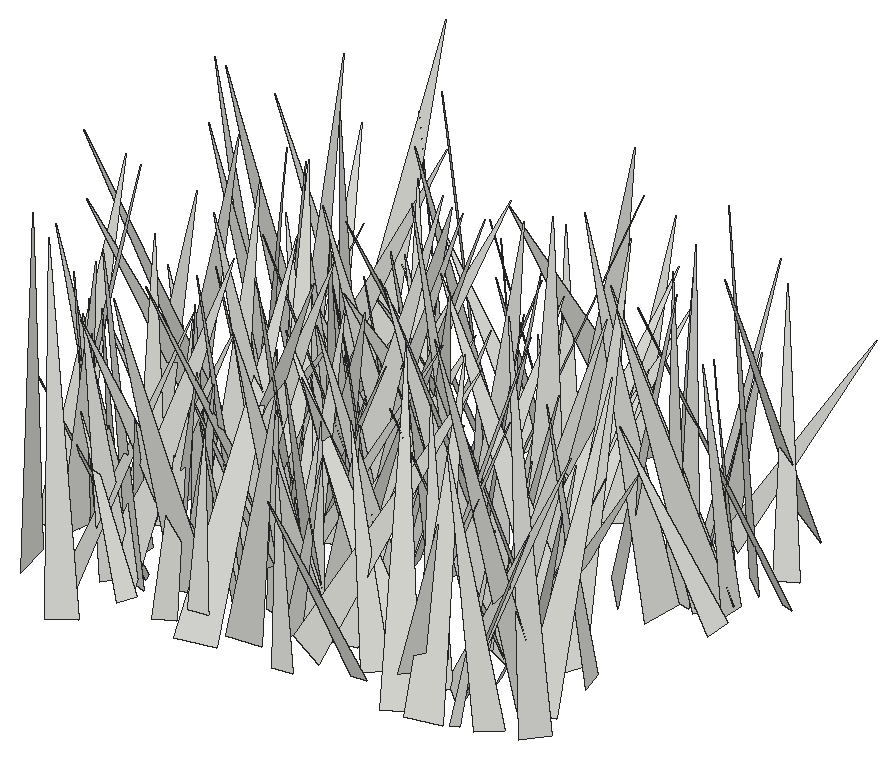
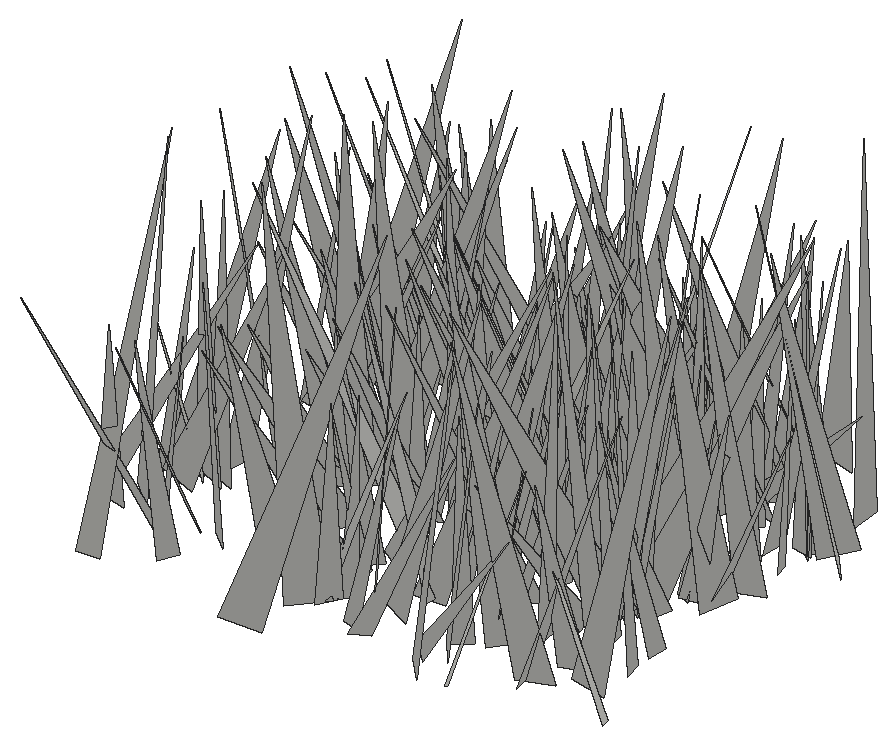
# SketchUp Ruby script. Lengths in inches.
U = 1.inch
M = Sketchup.active_model
def pt(a) = Geom::Point3d.new(a.map { |v| v * U })
def face(e, loops, mat)
  f = e.add_face(loops[0].map { |a| pt(a) })
  loops[1..].each { |l| e.add_face(l.map { |a| pt(a) }).erase! }
  f.material = f.back_material = mat if mat
  f
end
# faces: each face lists its corners as indices into pts; further lists are holes
def faces(e, pts, list, mat = nil) = list.each { |f| face(e, (f[0].is_a?(Array) ? f : [f]).map { |l| l.map { |i| pts[i] } }, mat) }
# xy, xz, yz: faces in a plane at the given z, y or x. An outline is a flat list of corners, or four numbers for a rectangle; further outlines are holes
def ring(l) = l.size == 4 ? [[l[0], l[1]], [l[2], l[1]], [l[2], l[3]], [l[0], l[3]]] : l.each_slice(2).to_a
def flat(e, list, mat, &to3) = list.each { |f| face(e, (f[0].is_a?(Array) ? f : [f]).map { |l| ring(l).map { |u, v| to3.(u, v) } }, mat) }
def xy(e, z, list, mat = nil) = flat(e, list, mat) { |x, y| [x, y, z] }
def xz(e, y, list, mat = nil) = flat(e, list, mat) { |x, z| [x, y, z] }
def yz(e, x, list, mat = nil) = flat(e, list, mat) { |y, z| [x, y, z] }
def lines(e, pts, list) = list.each { |a, b| e.add_line(pt(pts[a]), pt(pts[b])) }
# prism: a flat outline (further loops are holes) pulled along v
def prism(e, loops, v, mat = nil)
  f = face(e, loops, mat); d = Geom::Vector3d.new(v.map { |x| x * U })
  f.pushpull(f.normal.samedirection?(d) ? d.length : -d.length)
end
def box(e, o, s, mat = nil) = prism(e, [[o, [o[0] + s[0], o[1], o[2]], [o[0] + s[0], o[1] + s[1], o[2]], [o[0], o[1] + s[1], o[2]]]], [0, 0, s[2]], mat)
def at(x, y, z, deg = 0) = Geom::Transformation.translation(pt([x, y, z])) * Geom::Transformation.rotation(ORIGIN, Z_AXIS, deg.degrees)
def axes(o, x, y, z) = Geom::Transformation.new([*x, 0, *y, 0, *z, 0, *pt(o).to_a, 1])
def part(name) = M.definitions.add(name)
# library, detail: a bought-in or finely detailed component or shape, given as its bounding box
def library(name, o, s) = part(name).tap { |d| box(d.entities, o, s) }
def detail(e, o, s) = box(e.add_group.entities, o, s)
def put(e, d, t, mat = nil) = e.add_instance(d, t).tap { |i| i.material = mat if mat }
def group(e, t, mat = nil) = e.add_group.tap { |g| g.transformation = t; g.material = mat if mat }.entities
root = M.entities
c1 = part("fur_instance\#9")
p = [[0.8125,0,1.79],[0.67,-0.02,1.48],[0,-0.11,0],[0,0.11,0]]
faces(c1.entities,p,[[0,1,2,3]])
put(root,c1,axes([105.45,343.01,-27.1],[-1.01525,-4.25558,0.24661],[-4.20456,0.95799,-0.77812],[-0.70176,0.41691,4.30525]))
put(root,c1,axes([100.4375,342.52,-27.1],[2.54415,-5.74451,1.38415],[-5.89364,-2.3587,1.04378],[0.42454,1.68081,6.19537]))
put(root,c1,axes([94.2,339.64,-27.1],[-0.66678,7.09806,0.59701],[6.83624,0.46921,2.05647],[-2.00116,-0.76214,6.82627]))
put(root,c1,axes([102.92,341.7,-27.1],[-0.42877,3.87256,1.55947],[4.17346,0.35848,0.25729],[-0.1042,-1.57711,3.88772]))
put(root,c1,axes([90.58,342.37,-27.1],[7.19679,1.10507,2.93039],[1.40985,-7.70082,-0.55845],[-2.79655,-1.03845,7.25969]))
put(root,c1,axes([107.81,342.85,-27.1],[2.67886,-4.09104,0.57639],[-4.11516,-2.58128,0.80469],[0.36641,0.91951,4.82342]))
put(root,c1,axes([98.91,341.69,-27.1],[-3.06481,2.41196,1.362],[2.48233,3.29293,-0.24563],[1.22908,-0.63618,3.89234]))
put(root,c1,axes([96.72,344.24,-27.1],[1.44091,-6.85532,1.40735],[-6.89305,-1.6385,-0.92385],[-1.20912,1.1714,6.94393]))
put(root,c1,axes([95.12,342.3,-27.1],[-3.33504,1.53851,0.16438],[1.54705,3.32218,0.29368],[0.02564,-0.33558,3.66104]))
put(root,c1,axes([93.9,343.26,-27.1],[3.52477,-3.78027,2.43443],[-3.94318,-4.08529,-0.63451],[-2.1606,1.28874,5.1295]))
put(root,c1,axes([101.61,344.98,-27.1],[2.47706,-6.70826,1.39737],[-6.69174,-2.68793,-1.04158],[-1.47445,0.92925,7.07472]))
put(root,c1,axes([111.7,342.9,-27.1],[-2.10663,5.00928,1.58804],[5.23429,1.84857,1.1125],[-0.46582,-1.88217,5.31913]))
put(root,c1,axes([96.63,345.06,-27.1],[1.14957,-5.99203,1.40359],[-5.68779,-1.57972,-2.08556],[-2.35023,0.89221,5.73379]))
put(root,c1,axes([92.61,342.17,-27.1],[3.5807,5.01538,0.32607],[5.01642,-3.54168,-0.61141],[0.30977,-0.61982,6.13202]))
put(root,c1,axes([101.18,345.96,-27.1],[-2.08812,-6.42397,1.05341],[-6.15561,2.30841,1.87538],[2.11792,0.37569,6.48927]))
put(root,c1,axes([109.32,341.97,-27.1],[-1.91608,6.79372,1.10059],[6.8739,1.94553,-0.04218],[0.33984,-1.04766,7.05863]))
put(root,c1,axes([108.16,342.05,-27.1],[-2.69969,6.39263,0.77147],[6.43614,2.65406,0.5304],[-0.19237,-0.91623,6.91901]))
put(root,c1,axes([93.44,345.32,-27.1],[4.01305,-1.4697,0.35123],[-1.33059,-3.90931,-1.15533],[-0.71618,-0.97223,4.11458]))
put(root,c1,axes([94.71,343.38,-27.1],[-3.5063,-5.04513,2.56803],[-5.65565,3.25438,-1.32851],[0.24851,2.88062,5.99854]))
put(root,c1,axes([101.58,343.97,-27.1],[3.83893,-0.81047,1.08867],[-0.8917,-3.9684,0.19003],[-1.0232,0.41758,3.91895]))
put(root,c1,axes([109.6,343.875,-27.1],[4.10602,0.97464,0.35289],[0.9844,-4.11806,-0.08026],[-0.32469,-0.15985,4.21935]))
put(root,c1,axes([112.16,344.88,-27.1],[-1.47229,-7.46087,2.3597],[-7.72207,0.99683,-1.66627],[-1.2659,2.59656,7.41996]))
put(root,c1,axes([99.125,343.92,-27.1],[0.98464,3.25356,1.70885],[3.23357,-1.6077,1.19779],[-1.74639,-1.14237,3.18127]))
put(root,c1,axes([106.38,344.59,-27.1],[5.98331,3.57339,0.75673],[3.63565,-5.68637,-1.89446],[0.35186,-2.00943,6.70672]))
put(root,c1,axes([110.46,342.42,-27.1],[1.53322,3.39,0.04746],[3.12816,-1.43461,1.41479],[-1.30727,0.54307,3.44111]))
put(root,c1,axes([97.125,342,-27.1],[-5.33411,1.7362,0.45715],[1.45522,5.02033,-2.08679],[1.05153,1.85957,5.20696]))
put(root,c1,axes([108.97,344.19,-27.1],[3.86219,5.07234,0.99731],[5.04282,-3.42294,-2.11973],[1.1372,-2.04809,6.01264]))
put(root,c1,axes([105.66,343.76,-27.1],[-2.79772,3.91125,0.86225],[4.00509,2.73873,0.57209],[0.02536,-1.03446,4.77471]))
put(root,c1,axes([93.96,343.125,-27.1],[-0.17372,7.00266,1.70424],[6.95108,0.61311,-1.81067],[1.90374,-1.5996,6.76675]))
put(root,c1,axes([94.68,344.08,-27.1],[-3.03964,-3.22245,0.08473],[-2.53096,2.3136,-2.80576],[-1.9964,1.97328,3.42802]))
put(root,c1,axes([90.39,345.17,-27.1],[5.9168,-1.45412,1.7202],[-1.44139,-6.15974,-0.24915],[-1.73089,0.15879,6.08776]))
put(root,c1,axes([94.91,345.29,-27.1],[4.77554,-0.30271,1.03368],[-0.19329,-4.86277,-0.53104],[-1.0596,-0.47722,4.75556]))
put(root,c1,axes([108.18,344.16,-27.1],[2.13883,-4.28297,3.06723],[-5.00629,-2.68295,-0.2554],[-1.63976,2.60467,4.7805]))
put(root,c1,axes([108.15,344.68,-27.1],[3.13012,3.09581,1.75638],[3.35561,-3.34662,-0.08138],[-1.18695,-1.29717,4.40172]))
put(root,c1,axes([97.67,348.37,-27.1],[-5.6893,-5.57398,0.54513],[-5.22917,5.56506,2.3282],[2.00554,-1.30211,7.61688]))
put(root,c1,axes([102.64,343.47,-27.1],[1.86343,6.88556,0.79652],[6.51007,-1.45535,-2.64927],[2.37997,-1.41024,6.62304]))
put(root,c1,axes([90.87,345.73,-27.1],[-1.22041,-5.00142,1.71972],[-5.19067,1.47111,0.5948],[1.01418,1.51086,5.11369]))
put(root,c1,axes([102.03,344.65,-27.1],[3.56835,-1.26097,2.05366],[-1.59686,-3.9854,0.32755],[-1.80488,1.03305,3.77039]))
put(root,c1,axes([90.8,345.67,-27.1],[-3.25997,-4.21096,1.97124],[-4.4396,3.53441,0.20814],[1.38129,1.42168,5.3213]))
put(root,c1,axes([99.1,341.35,-27.1],[-6.13074,4.86156,0.06985],[4.48302,5.69573,-2.94734],[1.88206,2.26926,7.24803]))
put(root,c1,axes([100.23,345.47,-27.1],[-2.15609,-3.98258,0.83043],[-3.73233,1.56246,-2.1972],[-1.61872,1.70208,3.96005]))
put(root,c1,axes([93.35,344.57,-27.1],[2.79379,4.96818,0.70977],[4.95175,-2.59669,-1.31495],[0.8165,-1.25148,5.54607]))
put(root,c1,axes([91.86,346.13,-27.1],[-6.39617,-0.72322,1.67284],[-0.5993,6.59982,0.56183],[1.72113,-0.38959,6.41236]))
put(root,c1,axes([107.12,343.62,-27.1],[5.77926,4.78065,0.80242],[4.74367,-5.8345,0.5954],[-0.99801,-0.04845,7.47663]))
put(root,c1,axes([95.08,346.52,-27.1],[3.8804,-2.67072,0.47699],[-2.66948,-3.90717,-0.15997],[-0.48385,0.13783,4.70793]))
put(root,c1,axes([97.56,346.22,-27.1],[-5.57513,-2.9786,1.92177],[-3.03694,5.86084,0.2736],[1.82819,0.65252,6.315]))
put(root,c1,axes([106.45,344.64,-27.1],[-3.37764,5.82202,0.02709],[5.22944,3.02002,2.9728],[-2.55923,-1.51283,6.03878]))
put(root,c1,axes([113.3,343.6,-27.1],[-7.7657,1.30292,0.44128],[1.14319,7.51969,-2.08465],[0.76515,1.98873,7.59328]))
put(root,c1,axes([99.93,344.89,-27.1],[1.9045,4.44389,1.45881],[4.34306,-2.26488,1.22946],[-1.73613,-0.79091,4.67587]))
put(root,c1,axes([103.48,344.67,-27.1],[-2.78361,3.37072,1.19614],[3.02117,3.0272,-1.49988],[1.91443,0.12385,4.10617]))
put(root,c1,axes([94.83,347.07,-27.1],[-1.17903,-5.46423,1.73554],[-5.62366,1.44698,0.7353],[1.11548,1.51937,5.54141]))
put(root,c1,axes([108.22,347.99,-27.1],[-4.1053,-4.23157,0.31859],[-4.21802,4.11764,0.33835],[0.46467,-0.00766,5.88602]))
put(root,c1,axes([90.63,347.24,-27.1],[4.23333,1.58778,2.03705],[2.11026,-4.38143,-0.97034],[-1.48911,-1.69519,4.41595]))
put(root,c1,axes([99.28,346.92,-27.1],[1.07794,-7.21694,3.00432],[-7.53412,-1.768,-1.54384],[-2.08502,2.65746,7.13181]))
put(root,c1,axes([109.78,347.77,-27.1],[4.97063,-0.22915,0.23226],[-0.15729,-4.7897,-1.3593],[-0.28585,-1.34904,4.78665]))
put(root,c1,axes([89.03,345.81,-27.1],[-4.56158,-4.36485,4.54967],[-5.17144,5.80258,0.38189],[3.60662,2.79958,6.30192]))
put(root,c1,axes([100.9375,347.31,-27.1],[2.11868,-4.0714,0.72457],[-4.11944,-2.00647,0.77101],[0.3627,0.99394,4.52445]))
put(root,c1,axes([96.38,345.97,-27.1],[3.6811,-6.05089,2.6185],[-6.53456,-2.94932,2.37094],[0.87715,3.42178,6.67401]))
put(root,c1,axes([95.3,347.36,-27.1],[6.73019,-3.63445,0.24466],[-3.63894,-6.68481,0.79754],[0.16506,0.81773,7.60715]))
put(root,c1,axes([104.01,347.36,-27.1],[-0.12405,-5.8754,2.10648],[-6.00776,-0.4589,-1.63376],[-1.69244,2.05962,5.64504]))
put(root,c1,axes([89.72,344.99,-27.1],[-4.86903,5.31705,1.90275],[5.12727,5.21523,-1.45307],[2.36698,-0.35954,7.06166]))
put(root,c1,axes([100.45,345.7,-27.1],[-4.55508,3.55475,2.05706],[3.40532,4.98624,-1.07596],[2.29598,-0.34303,5.67691]))
put(root,c1,axes([97.7,349.18,-27.1],[-3.32814,-6.39102,1.50803],[-6.07577,3.63841,2.01068],[2.49085,0.3356,6.91945]))
put(root,c1,axes([100.39,350.08,-27.1],[5.08436,-3.96797,0.13679],[-3.71243,-4.83007,-2.12193],[-1.40762,-1.5937,6.0904]))
put(root,c1,axes([107.71,348.32,-27.1],[2.58278,-6.81445,2.81399],[-6.72051,-3.40212,-2.07037],[-3.03151,1.73634,6.98721]))
put(root,c1,axes([112.31,344.99,-27.1],[-4.09876,5.0884,1.14662],[4.86258,4.25523,-1.50159],[1.8873,0.0873,6.359]))
put(root,c1,axes([103.27,347.33,-27.1],[-3.89447,-3.70378,1.65585],[-4.00703,3.87088,-0.766],[0.63525,1.71028,5.3196]))
put(root,c1,axes([97.26,347.15,-27.1],[3.48145,-1.92251,0.90917],[-2.10367,-3.36896,0.93158],[-0.31179,1.26381,3.86636]))
put(root,c1,axes([109.67,345.94,-27.1],[4.18382,1.92252,0.07247],[1.86113,-4.08842,1.01327],[-0.48737,0.89131,4.49152]))
put(root,c1,axes([98.2,347.55,-27.1],[3.88099,1.49769,1.22771],[1.56049,-4.04689,0.00388],[-1.14683,-0.43823,4.15995]))
put(root,c1,axes([103.68,346.65,-27.1],[3.85077,0.95797,1.10657],[0.6489,-3.90916,1.12606],[-1.31192,0.87829,3.80501]))
put(root,c1,axes([112.32,348.13,-27.1],[-5.31437,-1.63311,1.48269],[-1.72892,5.48589,-0.1545],[1.36976,0.58821,5.55749]))
put(root,c1,axes([92.28,347.28,-27.1],[-1.52023,5.3398,1.43684],[5.52962,1.4775,0.35965],[0.03531,-1.48075,5.54032]))
put(root,c1,axes([109.75,348.72,-27.1],[-3.22494,-3.97651,0.65226],[-4.0077,3.07801,-1.05003],[-0.42001,1.16258,5.01102]))
put(root,c1,axes([110.79,346.65,-27.1],[-3.9364,0.91485,1.26316],[0.41585,3.92071,-1.54367],[1.50319,1.31107,3.73488]))
put(root,c1,axes([103.39,350.71,-27.1],[5.19652,-2.78136,0.42044],[-2.54268,-5.02221,-1.79688],[-1.20313,-1.39929,5.61347]))
put(root,c1,axes([92.28,349.21,-27.1],[3.64013,-0.49009,0.65042],[-0.33955,-3.62113,-0.82821],[-0.74023,-0.74902,3.57838]))
put(root,c1,axes([108.43,347.49,-27.1],[2.40948,7.1196,1.80641],[7.28749,-2.07931,-1.52526],[0.91887,-2.17835,7.35989]))
put(root,c1,axes([93.59,349.32,-27.1],[-2.68709,-2.60275,1.28992],[-2.48203,2.97011,0.82256],[1.50922,0.25052,3.6494]))
put(root,c1,axes([95.42,347.41,-27.1],[-1.01475,7.09695,1.79918],[7.31311,1.06925,-0.09303],[0.3496,-1.76734,7.16853]))
put(root,c1,axes([108.11,347.87,-27.1],[-3.37958,0.77927,1.41196],[0.41341,3.58754,-0.99047],[1.55884,0.73803,3.32382]))
put(root,c1,axes([105.96,351.17,-27.1],[-3.1075,-6.9448,0.74353],[-6.98342,3.07514,-0.46373],[-0.12218,0.86773,7.5942]))
put(root,c1,axes([111.23,348.48,-27.1],[-3.57057,6.8988,1.02898],[6.50769,2.8788,3.28081],[-2.51043,-2.34953,7.04122]))
put(root,c1,axes([93.41,351.46,-27.1],[0.03934,-7.1777,0.79174],[-6.87762,-0.27857,-2.18369],[-2.20103,0.74216,6.83757]))
put(root,c1,axes([95,350.375,-27.1],[-3.02685,-7.70536,1.30124],[-7.48247,2.45538,-2.86554],[-2.25353,2.19686,7.76679]))
put(root,c1,axes([90.37,349.37,-27.1],[0.14436,6.2225,2.72909],[6.68972,0.34776,-1.14678],[1.18962,-2.71069,6.11762]))
put(root,c1,axes([97.26,351.49,-27.1],[1.41766,-6.83451,0.48866],[-6.53171,-1.19719,2.20513],[2.07029,0.90294,6.62252]))
put(root,c1,axes([98.13,349.34,-27.1],[4.83025,3.81866,0.07193],[3.65702,-4.5907,-1.86288],[1.10161,-1.50398,5.86882]))
put(root,c1,axes([91.07,350.5,-27.1],[-3.67924,-0.76157,0.35539],[-0.68587,3.64327,0.70657],[0.48566,-0.62424,3.6902]))
put(root,c1,axes([108.58,349.42,-27.1],[4.05513,-1.76427,0.28786],[-1.75227,-3.78191,1.50543],[0.35366,1.49134,4.15818]))
put(root,c1,axes([100.34,350.86,-27.1],[-4.77204,-4.71706,0.72174],[-4.75307,4.60775,-1.31181],[-0.42413,1.43592,6.58044]))
put(root,c1,axes([97.88,349.22,-27.1],[4.13014,0.16234,0.60229],[0.00137,-4.03539,1.07832],[-0.62379,1.06603,3.99019]))
put(root,c1,axes([103.34,351.87,-27.1],[-1.39577,-4.42794,0.41329],[-4.44248,1.40819,0.08395],[0.20461,0.36877,4.64196]))
put(root,c1,axes([92.16,351.1,-27.1],[-1.43466,-3.23484,0.82707],[-3.31328,1.49057,0.08262],[0.41278,0.72144,3.53774]))
put(root,c1,axes([101.8,350.87,-27.1],[3.71055,0.76796,0.33165],[0.80764,-3.68168,-0.51076],[-0.21789,-0.56867,3.7546]))
put(root,c1,axes([97.42,351.26,-27.1],[3.61055,-0.61097,0.20103],[-0.59508,-3.6081,-0.27795],[-0.24409,-0.24103,3.65131]))
put(root,c1,axes([90.76,350.77,-27.1],[7.15421,-1.9799,2.12173],[-2.22149,-7.36827,0.61487],[-1.86728,1.18029,7.39761]))
put(root,c1,axes([99.53,351.57,-27.1],[-3.854,-0.48704,1.31581],[-0.33639,4.05498,0.51565],[1.36213,-0.37663,3.85028]))
put(root,c1,axes([93.33,352.4,-27.1],[3.21105,-3.45107,0.18225],[-3.45172,-3.21492,-0.06213],[-0.16965,0.09106,4.71348]))
put(root,c1,axes([105.21,349.98,-27.1],[4.98467,2.72403,1.68688],[2.57744,-5.26236,0.88159],[-1.90334,0.00786,5.61161]))
put(root,c1,axes([91.77,351.07,-27.1],[1.42744,-3.53628,2.17287],[-3.81125,-2.02664,-0.79456],[-1.64348,1.62839,3.72982]))
put(root,c1,axes([101.43,350.18,-27.1],[5.10289,-1.83511,1.25864],[-2.13691,-4.91957,1.49087],[-0.62081,1.84972,5.21387]))
put(root,c1,axes([92.49,352.96,-27.1],[3.64505,-0.39812,0.27738],[-0.20845,-3.18305,-1.82936],[-0.43816,-1.79764,3.17779]))
put(root,c1,axes([99.2,350.09,-27.1],[-0.29614,5.30233,1.4786],[4.87042,0.94241,-2.40408],[2.56516,-1.17721,4.73528]))
put(root,c1,axes([106.1,350.7,-27.1],[4.26152,0.65659,1.09682],[0.47447,-4.35714,0.76482],[-1.18701,0.6156,4.24343]))
put(root,c1,axes([100.08,354.11,-27.1],[-0.39765,-7.51588,0.89638],[-7.02687,0.7002,2.75371],[2.81337,0.68655,7.00455]))
put(root,c1,axes([96.21,353.125,-27.1],[6.38697,0.74513,2.00431],[1.2691,-6.40204,-1.66407],[-1.72101,-1.95564,6.21124]))
put(root,c1,axes([104.27,351.19,-27.1],[-7.25051,-1.24633,1.39987],[-1.43303,7.2913,-0.93068],[1.20805,1.16894,7.29774]))
put(root,c1,axes([110.76,348.75,-27.1],[0.70826,8.01559,0.32411],[7.89046,-0.75477,1.42384],[-1.44754,-0.19233,7.91985]))
put(root,c1,axes([92.92,353.05,-27.1],[-2.78076,-3.999,1.01738],[-3.97731,2.92434,0.62365],[1.09912,0.46468,4.83071]))
put(root,c1,axes([100.04,349.45,-27.1],[7.02888,1.27959,1.54515],[0.73768,-6.88381,2.34499],[-1.86566,2.099,6.7486]))
put(root,c1,axes([104.03,352.14,-27.1],[-3.12669,6.25889,3.83958],[6.87271,3.96367,-0.86451],[2.58493,-2.9678,6.9428]))
put(root,c1,axes([92.04,352.64,-27.1],[2.63596,-3.80697,0.02165],[-3.40971,-2.34911,2.07299],[1.69332,1.196,4.14053]))
put(root,c1,axes([96.32,350.53,-27.1],[-3.98192,5.65644,1.02142],[5.69703,4.04883,-0.21229],[0.76316,-0.7113,6.91418]))
put(root,c1,axes([106.88,352.08,-27.1],[4.92232,-5.34816,3.43981],[-5.97476,-5.37881,0.1869],[-2.17654,2.67018,7.26616]))
put(root,c1,axes([98.67,350.41,-27.1],[6.0321,-2.57805,3.10449],[-3.62742,-5.91038,2.14001],[-1.76807,3.33038,6.20104]))
put(root,c1,axes([102.83,353.49,-27.1],[3.43508,-2.31671,0.74566],[-2.27877,-3.51457,-0.42176],[-0.85461,0.05948,4.12177]))
put(root,c1,axes([99.67,353.32,-27.1],[0.21483,-6.37799,2.26736],[-6.52313,-0.80094,-1.63496],[-1.80789,2.13204,6.16862]))
put(root,c1,axes([96.33,351.8,-27.1],[-2.8304,4.89567,0.80261],[4.94903,2.72215,0.8485],[-0.34477,-1.11592,5.59096]))
put(root,c1,axes([98.75,352.76,-27.1],[-3.38469,-3.26483,1.22467],[-3.48648,3.19729,-1.11215],[0.05857,1.65326,4.56929]))
put(root,c1,axes([98.46,351.27,-27.1],[6.56769,-0.93589,1.93904],[-1.50422,-6.44796,1.98276],[-1.54048,2.30611,6.3308]))
put(root,c1,axes([113.5,354.08,-27.1],[-4.40105,0.97982,0.44244],[1.06612,4.21791,1.26401],[0.13855,-1.33202,4.328]))
put(root,c1,axes([96.5,353.11,-27.1],[-5.34365,-1.01248,1.41227],[-1.15776,5.47992,-0.452],[1.29585,0.72082,5.4199]))
put(root,c1,axes([108.83,353.86,-27.1],[5.37674,4.78999,2.15375],[5.23773,-5.117,-1.69543],[-0.38579,-2.71372,6.99849]))
put(root,c1,axes([112.45,355.13,-27.1],[3.31279,-6.01066,2.01721],[-5.81791,-3.7865,-1.72802],[-2.51972,0.84034,6.64203]))
put(root,c1,axes([93.4,354.22,-27.1],[-1.73003,-6.76572,2.01517],[-7.01807,1.42401,-1.24409],[-0.76325,2.2419,6.8717]))
put(root,c1,axes([101.33,351.58,-27.1],[-5.19034,4.80556,0.45379],[4.78626,5.21014,-0.43029],[0.62529,0.00866,7.0603]))
put(root,c1,axes([111.18,353.71,-27.1],[-8.03417,0.61584,1.78735],[0.70083,8.21761,0.3188],[1.75577,-0.4621,8.05143]))
put(root,c1,axes([99.37,357.03,-27.1],[4.98513,-4.06782,0.78587],[-3.3159,-4.65458,-3.05875],[-2.48386,-1.95039,5.66063]))
put(root,c1,axes([103.35,353.07,-27.1],[-3.61899,-3.55384,3.43713],[-4.24844,4.41399,0.09065],[2.52873,2.32973,5.07136]))
put(root,c1,axes([102.11,355.68,-27.1],[-3.14306,-6.22127,0.26286],[-6.12359,3.03481,-1.39417],[-1.12913,0.859,6.8293]))
put(root,c1,axes([94.89,355.38,-27.1],[4.79188,-1.27621,1.00499],[-1.01396,-4.79557,-1.25507],[-1.26909,-0.98723,4.79746]))
put(root,c1,axes([107.52,352.19,-27.1],[-1.55041,4.4226,0.08121],[4.26043,1.51619,-1.23272],[1.18941,0.33394,4.52145]))
put(root,c1,axes([93.67,353.16,-27.1],[1.68916,7.29229,2.94864],[7.0223,-2.75681,2.79508],[-3.5439,-1.98689,6.94394]))
put(root,c1,axes([103.02,352.35,-27.1],[-0.26942,5.43204,0.24352],[5.36362,0.30555,-0.88154],[0.89325,-0.19629,5.36679]))
put(root,c1,axes([96.1875,356.01,-27.1],[-4.24869,-0.73201,1.00331],[-0.4187,4.21079,1.29914],[1.16925,-1.15205,4.11089]))
put(root,c1,axes([92.08,355.3,-27.1],[6.17707,1.48648,1.9777],[1.80034,-6.34915,-0.85095],[-1.69697,-1.32504,6.29616]))
put(root,c1,axes([90.29,354.93,-27.1],[4.64255,0.07182,0.51653],[0.0806,-4.67045,-0.07504],[-0.51523,-0.08349,4.6425]))
put(root,c1,axes([99.95,355.29,-27.1],[-3.61147,3.35043,1.62323],[3.67501,3.56996,0.80783],[0.59541,-1.71259,4.85958]))
put(root,c1,axes([111.03,354.77,-27.1],[1.52535,6.05061,2.3847],[6.37233,-1.8801,0.69429],[-1.30004,-2.1163,6.20117]))
put(root,c1,axes([113.08,355.4,-27.1],[-4.88413,-0.13594,1.40409],[-0.16648,5.08029,-0.08723],[1.4008,0.12978,4.88524]))
put(root,c1,axes([90.17,356.54,-27.1],[6.17791,2.14602,1.95241],[2.61385,-6.11017,-1.55482],[-1.25898,-2.15507,6.35252]))
put(root,c1,axes([96.7,356.21,-27.1],[-3.36264,-2.39418,1.21792],[-2.41208,3.55006,0.31902],[1.18208,0.43333,4.11555]))
put(root,c1,axes([102.39,354.14,-27.1],[7.40183,3.33475,0.3809],[3.31775,-7.40888,0.39208],[-0.5081,0.20159,8.10888]))
put(root,c1,axes([102.61,356.28,-27.1],[1.94389,-4.04886,0.80465],[-4.08173,-1.75236,1.04312],[0.61659,1.16421,4.36851]))
put(root,c1,axes([112.21,355.78,-27.1],[-0.7555,-5.85213,2.53673],[-5.87032,-0.36099,-2.58111],[-2.49433,2.62211,5.30623]))
put(root,c1,axes([111.65,354.98,-27.1],[2.95559,2.2846,0.71516],[2.24296,-3.03986,0.44126],[-0.83663,-0.07885,3.70947]))
put(root,c1,axes([93.08,353.83,-27.1],[6.18283,-3.26103,2.17206],[-3.91127,-5.37775,3.05962],[-0.2327,3.74499,6.28493]))
put(root,c1,axes([95.04,357.83,-27.1],[3.43044,-6.71204,0.2285],[-6.5076,-3.25868,1.97581],[1.6598,1.09595,7.27431]))
put(root,c1,axes([99.24,356.86,-27.1],[6.07626,0.90493,0.17774],[0.92213,-5.94508,-1.25588],[0.01299,-1.26833,6.01354]))
put(root,c1,axes([98.6,355.93,-27.1],[-2.6227,-3.62693,1.52989],[-3.9333,2.34177,-1.19122],[-0.15598,1.93268,4.31442]))
put(root,c1,axes([92.86,355.29,-27.1],[2.51079,7.35519,2.45383],[7.71335,-2.63218,-0.00261],[-0.79014,-2.32314,7.77193]))
put(root,c1,axes([96.17,354.79,-27.1],[1.82211,6.46965,0.85286],[6.26515,-1.48669,-2.10749],[1.8253,-1.35544,6.38239]))
put(root,c1,axes([111.45,354.9,-27.1],[1.52535,6.57132,1.88983],[6.63248,-1.89273,1.22809],[-1.66251,-1.52175,6.63331]))
put(root,c1,axes([94.18,356.625,-27.1],[-6.46976,-1.55499,2.98827],[-1.52534,7.12153,0.40334],[3.00351,0.26714,6.64177]))
put(root,c1,axes([114.45,356.99,-27.1],[-3.99389,-5.07881,0.29207],[-4.86869,3.70838,-2.09153],[-1.47493,1.51142,6.11318]))
put(root,c1,axes([93.76,354.77,-27.1],[3.8069,0.05751,0.20355],[-0.0416,-3.39391,1.73693],[-0.20739,1.73647,3.38805]))
put(root,c1,axes([101.64,357.31,-27.1],[-4.27511,-3.26782,2.05551],[-3.38668,4.64678,0.34365],[1.85313,0.95347,5.37002]))
put(root,c1,axes([90.7,358.55,-27.1],[-1.04582,-7.4675,1.55674],[-7.62212,0.96116,-0.50998],[-0.30029,1.61039,7.52311]))
put(root,c1,axes([105.11,354.59,-27.1],[-2.16647,5.60636,0.16983],[5.26617,2.09582,-2.00715],[1.93067,0.57445,5.66535]))
put(root,c1,axes([112.53,357.44,-27.1],[-4.94486,-5.49387,2.91837],[-6.02867,5.15162,-0.51692],[1.53451,2.53562,7.37341]))
put(root,c1,axes([96.35,358.8,-27.1],[1.68114,-3.92704,0.2758],[-3.91607,-1.63754,0.5539],[0.40264,0.46985,4.23569]))
put(root,c1,axes([99.78,358.54,-27.1],[-2.51805,-6.35566,1.6356],[-6.55451,2.34778,-0.96776],[-0.32873,1.87181,6.76746]))
put(root,c1,axes([101.77,358.78,-27.1],[3.2467,-2.02133,0.75684],[-1.94033,-3.33216,-0.57574],[-0.94537,-0.10279,3.78092]))
put(root,c1,axes([102.22,357.1875,-27.1],[3.63401,0.67625,1.41653],[0.37628,-3.84346,0.86953],[-1.5239,0.6636,3.59267]))
put(root,c1,axes([104.33,356.34,-27.1],[-1.05033,5.0969,0.69056],[4.61293,1.24522,-2.17458],[2.27512,-0.17172,4.72788]))
put(root,c1,axes([110.62,358.54,-27.1],[-2.70575,-2.79772,1.42447],[-3.05403,2.78134,-0.3384],[0.7275,1.27058,3.87735]))
put(root,c1,axes([111.27,362.21,-27.1],[-2.73458,-7.67612,0.26637],[-7.34259,2.69559,2.30041],[2.25392,-0.53168,7.81722]))
put(root,c1,axes([108.17,358.37,-27.1],[3.30572,4.13092,2.03155],[4.38871,-3.58299,0.14433],[-1.38957,-1.489,5.28881]))
put(root,c1,axes([102.8,358.68,-27.1],[-4.27144,-3.27285,0.83505],[-3.36103,3.98484,-1.57435],[-0.33515,1.75031,5.14569]))
put(root,c1,axes([92.85,359.51,-27.1],[-6.22564,-1.43503,0.72375],[-1.44178,6.26598,0.02194],[0.71021,0.14105,6.38885]))
put(root,c1,axes([103.62,362.82,-27.1],[3.75973,-6.87339,0.18092],[-6.4988,-3.61971,-2.46477],[-2.2454,-1.03249,7.43666]))
put(root,c1,axes([94.85,361.65,-27.1],[-2.93741,-3.09466,0.01129],[-2.71699,2.58635,2.03327],[1.48156,-1.39259,3.75115]))
put(root,c1,axes([100.41,360.34,-27.1],[-1.40933,-4.17013,0.64925],[-4.20295,1.44894,0.18319],[0.38311,0.55526,4.39803]))
put(root,c1,axes([102.68,359.98,-27.1],[5.49312,-5.94068,1.74056],[-6.16398,-5.4638,0.80479],[-0.57141,1.8305,8.05098]))
put(root,c1,axes([105.65,358.01,-27.1],[-4.4871,3.83069,1.41429],[3.5666,4.69982,-1.41404],[1.98841,0.2144,5.72789]))
put(root,c1,axes([91.99,357.76,-27.1],[-1.75814,5.2069,0.13379],[5.20853,1.75836,0.01288],[0.0306,-0.13088,5.4957]))
put(root,c1,axes([88.56,360.1875,-27.1],[3.77978,1.93812,0.15141],[1.88384,-3.56988,-1.33157],[0.48001,-1.25124,4.0336]))
put(root,c1,axes([99.75,360.64,-27.1],[-4.14397,2.00475,0.46664],[2.04964,3.92263,1.34951],[-0.1891,-1.41534,4.40117]))
put(root,c1,axes([102.18,359.42,-27.1],[-4.07522,2.66076,1.05763],[2.66001,4.19896,-0.31421],[1.05952,-0.30776,4.85678]))
put(root,c1,axes([108.82,360.55,-27.1],[3.79566,-1.87078,0.73995],[-1.92959,-3.83243,0.2087],[-0.56925,0.51676,4.2265]))
put(root,c1,axes([96.5,359.53,-27.1],[3.70498,4.05955,2.96614],[3.93602,-4.63444,1.42637],[-3.1282,-1.02317,5.30776]))
put(root,c1,axes([113.22,358.46,-27.1],[-0.43332,5.55714,0.38235],[5.39105,0.32188,1.43136],[-1.40165,-0.47995,5.3871]))
put(root,c1,axes([97.22,360.25,-27.1],[-2.6027,-3.00196,0.39616],[-2.70686,2.07255,-2.07851],[-1.35707,1.62343,3.38609]))
put(root,c1,axes([109.84,357.76,-27.1],[2.78013,5.13783,0.11647],[4.85085,-2.66723,1.86951],[-1.69707,0.79284,5.53456]))
put(root,c1,axes([109.74,359.6,-27.1],[2.70061,4.81345,0.08968],[4.52857,-2.505,-1.92033],[1.63383,-1.01307,5.17446]))
put(root,c1,axes([96.54,361.39,-27.1],[-4.69837,-4.55111,2.1601],[-4.81656,4.92378,-0.10244],[1.47629,1.58022,6.5404]))
put(root,c1,axes([92.45,359.45,-27.1],[-1.03239,7.59334,1.92082],[7.72051,1.31303,-1.04105],[1.31985,-1.74108,7.59215]))
